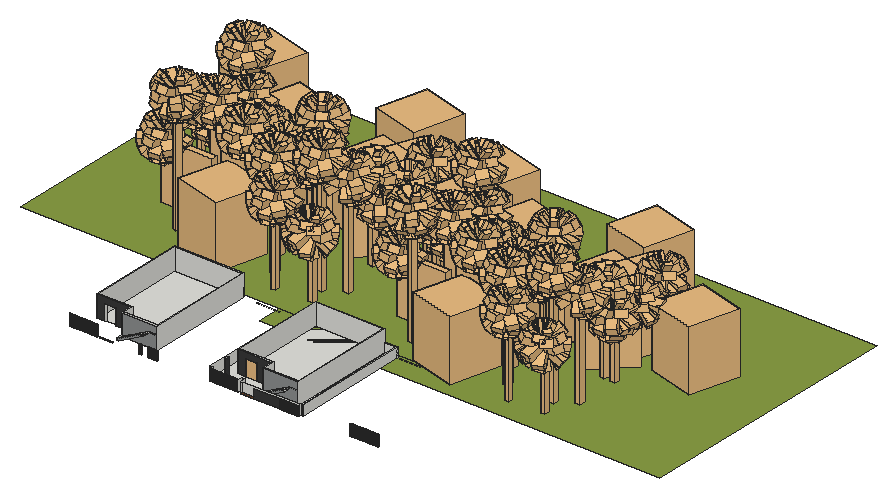
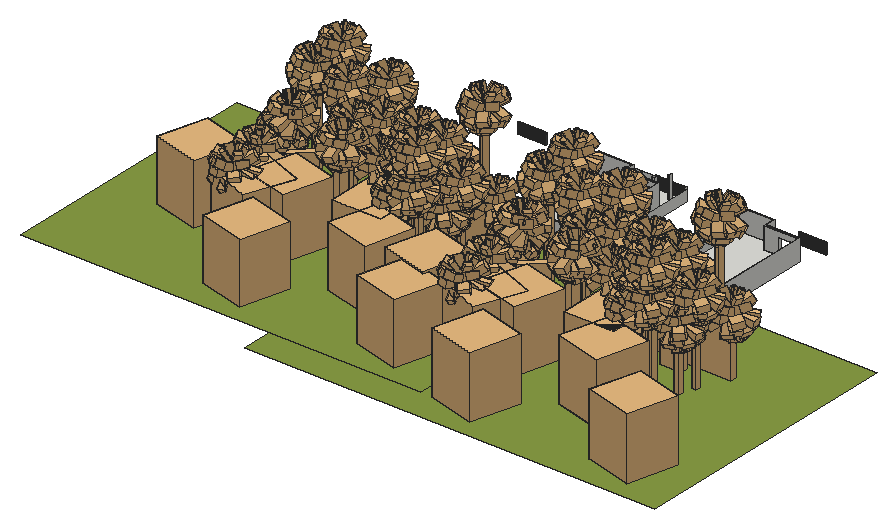
# SketchUp Ruby script. Lengths in inches.
U = 1.inch
M = Sketchup.active_model
def pt(a) = Geom::Point3d.new(a.map { |v| v * U })
def face(e, loops, mat)
  f = e.add_face(loops[0].map { |a| pt(a) })
  loops[1..].each { |l| e.add_face(l.map { |a| pt(a) }).erase! }
  f.material = f.back_material = mat if mat
  f
end
# faces: each face lists its corners as indices into pts; further lists are holes
def faces(e, pts, list, mat = nil) = list.each { |f| face(e, (f[0].is_a?(Array) ? f : [f]).map { |l| l.map { |i| pts[i] } }, mat) }
# xy, xz, yz: faces in a plane at the given z, y or x. An outline is a flat list of corners, or four numbers for a rectangle; further outlines are holes
def ring(l) = l.size == 4 ? [[l[0], l[1]], [l[2], l[1]], [l[2], l[3]], [l[0], l[3]]] : l.each_slice(2).to_a
def flat(e, list, mat, &to3) = list.each { |f| face(e, (f[0].is_a?(Array) ? f : [f]).map { |l| ring(l).map { |u, v| to3.(u, v) } }, mat) }
def xy(e, z, list, mat = nil) = flat(e, list, mat) { |x, y| [x, y, z] }
def xz(e, y, list, mat = nil) = flat(e, list, mat) { |x, z| [x, y, z] }
def yz(e, x, list, mat = nil) = flat(e, list, mat) { |y, z| [x, y, z] }
def lines(e, pts, list) = list.each { |a, b| e.add_line(pt(pts[a]), pt(pts[b])) }
# prism: a flat outline (further loops are holes) pulled along v
def prism(e, loops, v, mat = nil)
  f = face(e, loops, mat); d = Geom::Vector3d.new(v.map { |x| x * U })
  f.pushpull(f.normal.samedirection?(d) ? d.length : -d.length)
end
def box(e, o, s, mat = nil) = prism(e, [[o, [o[0] + s[0], o[1], o[2]], [o[0] + s[0], o[1] + s[1], o[2]], [o[0], o[1] + s[1], o[2]]]], [0, 0, s[2]], mat)
def at(x, y, z, deg = 0) = Geom::Transformation.translation(pt([x, y, z])) * Geom::Transformation.rotation(ORIGIN, Z_AXIS, deg.degrees)
def axes(o, x, y, z) = Geom::Transformation.new([*x, 0, *y, 0, *z, 0, *pt(o).to_a, 1])
def part(name) = M.definitions.add(name)
# library, detail: a bought-in or finely detailed component or shape, given as its bounding box
def library(name, o, s) = part(name).tap { |d| box(d.entities, o, s) }
def detail(e, o, s) = box(e.add_group.entities, o, s)
def put(e, d, t, mat = nil) = e.add_instance(d, t).tap { |i| i.material = mat if mat }
def group(e, t, mat = nil) = e.add_group.tap { |g| g.transformation = t; g.material = mat if mat }.entities
root = M.entities
M.materials.add("48,62,1").color = [75, 79, 82]
M.materials.add("COCOLUMBER1").color = [119, 109, 95]
M.materials.add("[Blacktop Old 02]").color = [143, 145, 145]
M.materials.add("[Color M07]").color = [58, 58, 58]
M.materials.add("[Grass Light Green]").color = [138, 158, 69]
M.materials.add("[Stone_Flagstone_Ashlar]").color = [175, 116, 102]
M.materials.add("[Wood Veneer 01]").color = [120, 70, 37]
M.materials.add("hpl-fundermax-sheets-500x500").color = [131, 93, 58]
c1 = part("Group\#60")
prism(c1.entities,[[[-0.75,0,69],[-0.75,0,68],[-0.75,-1.375,68],[-0.75,-1.375,4],[-0.75,0,4],[-0.75,0,3],[-0.75,-2.75,3],[-0.75,-2.75,69]]],[1.5,0,0])
c2 = part("Group\#59")
box(c2.entities,[0,-0.75,0],[0.75,0.75,72])
c3 = part("Group\#78")
xy(c3.entities,0,[[4.5,0,61.75,2],[62.25,0,120,2]])
xy(c3.entities,72,[[4.5,0,61.75,2],[62.25,0,120,2]])
xz(c3.entities,0,[[4.5,0,53.25,72],[54,0,57,72],[57.75,0,61.75,72],[62.25,0,66.25,72],[67,0,120,72]])
xz(c3.entities,0,[[57,0,57.75,72],[66.25,0,67,72]],"48,62,1")
xz(c3.entities,2,[[4.5,0,61.75,72],[62.25,0,120,72]])
yz(c3.entities,4.5,[[0,0,2,72]])
yz(c3.entities,61.75,[[0,0,2,72]])
yz(c3.entities,62.25,[[0,0,2,72]])
yz(c3.entities,120,[[0,0,2,72]])
put(c3.entities,c1,at(58,0,0))
put(c3.entities,c1,at(66,0,0))
put(c3.entities,c2,at(53.25,0,0),"48,62,1")
put(c3.entities,c2,at(49.5,0,0),"48,62,1")
put(c3.entities,c2,at(45.75,0,0),"48,62,1")
put(c3.entities,c2,at(42,0,0),"48,62,1")
put(c3.entities,c2,at(38.25,0,0),"48,62,1")
put(c3.entities,c2,at(34.5,0,0),"48,62,1")
put(c3.entities,c2,at(30.75,0,0),"48,62,1")
put(c3.entities,c2,at(27,0,0),"48,62,1")
put(c3.entities,c2,at(23.25,0,0),"48,62,1")
put(c3.entities,c2,at(19.5,0,0),"48,62,1")
put(c3.entities,c2,at(15.75,0,0),"48,62,1")
put(c3.entities,c2,at(12,0,0),"48,62,1")
put(c3.entities,c2,at(8.25,0,0),"48,62,1")
put(c3.entities,c2,at(4.5,0,0),"48,62,1")
put(c3.entities,c2,at(70,0,0),"48,62,1")
put(c3.entities,c2,at(73.75,0,0),"48,62,1")
put(c3.entities,c2,at(77.5,0,0),"48,62,1")
put(c3.entities,c2,at(81.25,0,0),"48,62,1")
put(c3.entities,c2,at(85,0,0),"48,62,1")
put(c3.entities,c2,at(88.75,0,0),"48,62,1")
put(c3.entities,c2,at(92.5,0,0),"48,62,1")
put(c3.entities,c2,at(96.25,0,0),"48,62,1")
put(c3.entities,c2,at(100,0,0),"48,62,1")
put(c3.entities,c2,at(103.75,0,0),"48,62,1")
put(c3.entities,c2,at(107.5,0,0),"48,62,1")
put(c3.entities,c2,at(111.25,0,0),"48,62,1")
put(c3.entities,c2,at(115,0,0),"48,62,1")
put(c3.entities,c2,at(119.25,0,0),"48,62,1")
c4 = library("door (1)",[38.93,25.48,0],[40,9.94,82.68])
c5 = library("Palm frond \#1",[-21.27,-0.38,-4.44],[74.64,151.68,26.05])
c6 = part("Palm frond cluster")
put(c6.entities,c5,axes([98.98,59.12,-6.6],[-0.57786,0.81614,0],[-0.81614,-0.57786,0],[0,0,1.8876]))
put(c6.entities,c5,axes([105.83,88.13,9.87],[-0.67944,-0.73373,0],[0.7249,-0.67126,-0.15471],[0.21427,-0.19842,1.86487]))
put(c6.entities,c5,axes([73.46,76.73,-6.83],[1,0,0],[0,0.99443,-0.10543],[0,0.19901,1.87708]))
c7 = part("Palm tree")
put(c7.entities,c5,axes([108.09,116.23,112.23],[0.60444,0.79634,0.02211],[-0.38669,0.31755,-0.86581],[-0.57427,0.42444,0.41215]))
put(c7.entities,c5,axes([136.99,132.05,110.62],[-0.9152,-0.38852,0.10706],[0.08408,-0.44389,-0.89213],[0.32496,-0.66577,0.36188]))
put(c7.entities,c5,axes([122.18,113.8,111.54],[0.08804,0.99481,0.05098],[-0.50379,0.08862,-0.85927],[-0.70852,0.0412,0.41966]))
put(c7.entities,c5,axes([127.99,125.91,114.12],[-0.30715,0.21543,0.04369],[-0.00716,-0.23041,1.0858],[0.26841,0.36655,0.07955]))
put(c7.entities,c5,axes([103.59,126.54,118.32],[0.96893,0.24682,0.01605],[-0.22321,0.84461,0.48663],[0.20112,-0.89679,1.64874]))
put(c7.entities,c5,axes([132.625,118.58,110.86],[-0.79198,0.60227,0.10017],[-0.36651,-0.33776,-0.86694],[-0.4026,-0.59638,0.40255]))
put(c7.entities,c5,axes([132.69,143.375,115.86],[-0.48474,-0.87071,0.083],[0.68927,-0.43869,-0.5766],[1.01639,-0.4196,1.53425]))
put(c7.entities,c6,axes([128.89,9.89,132.21],[0.59014,0.791,-0.16144],[-0.79634,0.60321,0.04452],[0.1326,0.10229,0.98588]))
put(c7.entities,c5,axes([110.58,141.22,117.1],[0.63855,-0.76931,0.0202],[0.63758,0.51415,-0.57371],[0.8135,0.71582,1.54559]))
put(c7.entities,c5,axes([124.78,146.64,115.88],[-0.11221,-0.99112,0.07129],[0.92652,-0.13028,-0.35296],[0.67787,0.04993,1.76097]))
put(c7.entities,c5,axes([122.51,149.42,117.04],[0.39103,-0.91975,0.03404],[0.19966,0.04866,-0.97866],[0.74078,0.32113,0.1671]))
put(c7.entities,c5,axes([109.625,140.35,117.99],[0.86054,-0.50891,0.02211],[0.4462,0.77402,0.44921],[-0.46382,-0.71105,1.68592]))
put(c7.entities,c5,axes([116.71,128.1875,118.1],[0.61604,-0.07661,0.00027],[0.03235,0.25679,-0.96593],[0.09819,0.79033,0.2134]),"COCOLUMBER1")
put(c7.entities,c5,axes([106.79,121.78,118.63],[0.90526,0.41496,-0.09122],[-0.38356,0.70587,-0.59551],[-0.34491,1.08363,1.50659]))
put(c7.entities,c5,axes([127.38,115.49,111.15],[-0.41996,0.90406,0.07938],[-0.48716,-0.15078,-0.8602],[-0.63133,-0.32974,0.41534]))
put(c7.entities,c5,axes([126.87,112.82,117.51],[-0.39428,0.9188,-0.01857],[-0.74747,-0.33238,-0.57517],[-1.00919,-0.40185,1.54373]))
put(c7.entities,c5,axes([136.51,114.68,116.54],[-0.8132,0.57038,0.11567],[-0.44883,-0.74115,0.49924],[0.69933,0.66833,1.62089]))
put(c7.entities,c5,axes([139.34,132.85,114.96],[-0.95658,-0.27018,0.10937],[0.1925,-0.86734,-0.45898],[0.41314,-0.78901,1.66428]))
put(c7.entities,c5,axes([114.58,111.42,117.76],[0.273,0.96044,0.05495],[-0.82871,0.20578,0.52048],[0.92224,-0.35418,1.60843]))
put(c7.entities,c6,axes([34.06,50.17,99.19],[1,0,0],[0,0.96593,0.25882],[0,-0.25882,0.96593]))
put(c7.entities,c5,axes([129.57,143.93,113.7],[-0.59821,-0.79634,0.08934],[0.41703,-0.40458,-0.81388],[0.56418,-0.37071,0.47337]))
put(c7.entities,c5,axes([130.72,144.4375,116.95],[-0.38164,-0.91976,0.09155],[0.8496,-0.31006,0.42666],[-0.68716,0.45418,1.6984]))
put(c7.entities,c5,axes([131.04,111.78,119.35],[-0.80044,0.5994,0.00413],[-0.42618,-0.56425,-0.7071],[-0.79563,-1.07169,1.33472]))
put(c7.entities,c5,axes([110.2,144.05,126.35],[0.60643,-0.7943,0.03632],[0.64903,0.52087,0.55448],[-0.86705,-0.59022,1.56936]))
put(c7.entities,c5,axes([142.64,131.42,116.29],[-0.95847,-0.25692,0.12379],[0.28487,-0.84195,0.45823],[-0.02548,0.8956,1.66141]))
put(c7.entities,c5,axes([119.45,118.27,117.33],[0.21648,0.59293,0.03228],[-0.46829,0.12335,0.87492],[0.90601,-0.35995,0.53567]))
put(c7.entities,c5,axes([117.27,113.7,118.04],[0.23506,0.97049,-0.05375],[-0.80388,0.16302,-0.57201],[-1.03133,0.33537,1.54496]))
put(c7.entities,c5,axes([111.15,130.86,117.79],[0.59448,-0.21434,0.01115],[0.17045,0.51639,0.83922],[-0.32671,-0.8747,0.60458]))
put(c7.entities,c5,axes([131.22,120.64,116.67],[-0.51397,0.3605,0.07311],[-0.2051,-0.46687,0.86021],[0.60585,0.75173,0.55245]))
put(c7.entities,c5,axes([124.93,138.67,117.02],[-0.21153,-0.59293,0.0562],[0.56288,-0.12335,0.81728],[-0.84066,0.35995,0.63331]))
put(c7.entities,c5,axes([125.97,109.88,116.19],[-0.24621,0.96375,0.10281],[-0.94431,-0.21463,-0.24942],[-0.41209,-0.29916,1.81761]))
put(c7.entities,c5,axes([112.49,114.18,118.67],[0.68775,0.72163,-0.07906],[-0.67912,0.60109,-0.4213],[-0.48416,0.64828,1.70539]))
c8 = part("Group\#557")
put(c8.entities,c7,axes([-0.04,31.24,176.27],[0.54092,-0.14494,0],[0.14494,0.54092,0],[0,0,0.56]),"[Stone_Flagstone_Ashlar]")
g1 = group(c8.entities,at(43.85,611.85,9.84))
detail(g1,[29.01,-534.03,-9.84],[20.18,17.89,236.22])
c9 = library("Group\#544",[280.3,-607.43,-9.84],[21.76,21.76,393.7])
c10 = part("Group\#559")
put(c10.entities,c7,axes([14.65,13.97,332.76],[0.56,0,0],[0,0.56,0],[0,0,0.56]),"[Stone_Flagstone_Ashlar]")
put(c10.entities,c9,at(-205.96,691.71,9.84))
c11 = library("Group\#545",[336.49,-607.32,-9.84],[23.63,23.62,472.44])
c12 = part("Group\#558")
put(c12.entities,c7,axes([14.65,13.97,408.41],[0.56,0,0],[0,0.56,0],[0,0,0.56]),"[Stone_Flagstone_Ashlar]")
put(c12.entities,c11,axes([-199.25,630.26,9.84],[0.8099,0,0],[0,0.92,0],[0,0,1]))
c13 = part("Group\#555")
put(c13.entities,c7,axes([14.65,13.97,257.21],[0.56,0,0],[0,0.56,0],[0,0,0.56]),"[Stone_Flagstone_Ashlar]")
g2 = group(c13.entities,at(-87.26,634.75,9.84))
detail(g2,[163.83,-557.35,-9.84],[17.02,18.12,316.37])
c14 = library("Coconut",[0,0,0],[6,6,6])
c15 = part("Group\#543")
detail(c15.entities,[126.53,-566.4375,-31.76],[21.43,21.47,314.96])
c16 = part("Group\#554")
put(c16.entities,c7,axes([14.65,13.97,253.0625],[0.56,0,0],[0,0.56,0],[0,0,0.56]),"[Stone_Flagstone_Ashlar]")
put(c16.entities,c15,at(-54.86,642.08,31.76))
c17 = library("Group\#560",[-31.7,-22.28,0],[197.44,197.48,245.38])
c18 = library("Group\#550",[-86.05,-583.93,-9.84],[105.44,25.13,372.44])
c19 = part("Group\#562")
put(c19.entities,c7,axes([14.65,13.97,296.01],[0.56,0,0],[0,0.56,0],[0,0,0.56]),"[Stone_Flagstone_Ashlar]")
put(c19.entities,c18,axes([86.81,656.51,9.45],[1,0,0],[0,1,0],[0,0,0.96]))
c20 = library("Group\#553",[-509.61,-583,-9.84],[198.33,25,224.95])
c21 = part("Group\#561")
put(c21.entities,c7,axes([14.65,13.97,164.57],[0.56,0,0],[0,0.56,0],[0,0,0.56]),"[Stone_Flagstone_Ashlar]")
put(c21.entities,c20,at(588.97,655.37,9.84))
c22 = library("Group\#551",[-201.8,-584.81,-9.84],[84.72,26.88,386.61])
c23 = library("Group\#552",[-284.02,-582.12,-9.84],[34.81,21.51,275.59])
c24 = part("LANDSCAPING+Coconut+Trees")
xy(c24.entities,0,[[-341.57,-22.89,1280.875,1071.24]],"[Grass Light Green]")
put(c24.entities,c8,at(644.25,162.65,0.08,-90))
put(c24.entities,c10,at(534.68,153.22,0.24))
put(c24.entities,c12,at(627.57,68.88,0.24))
g3 = group(c24.entities,at(441.06,62.32,0.24))
put(g3,c7,axes([14.65,13.97,334.3],[0.56,0,0],[0,0.56,0],[0,0,0.56]),"[Stone_Flagstone_Ashlar]")
g4 = group(g3,at(-161.71,683.51,9.84))
detail(g4,[235.77,-605.36,-9.84],[21.85,21.73,393.32])
put(c24.entities,c13,at(507.45,-17.04,0.04))
g5 = group(c24.entities,at(384.92,163.75,0.52))
put(g5,c7,axes([14.65,13.97,253.0625],[0.56,0,0],[0,0.56,0],[0,0,0.56]),"[Stone_Flagstone_Ashlar]")
put(g5,c14,axes([78.15,82.49,296.44],[0.8993,1.53487,-0.03138],[-1.51998,0.89531,0.23158],[0.21557,-0.09025,1.76378]))
put(g5,c14,axes([79.68,82.54,287.24],[0.80142,1.36782,-0.02796],[-1.35455,0.79787,0.20637],[0.1921,-0.08042,1.57182]))
put(g5,c14,axes([77.51,71.8,291.02],[0.8993,1.53487,-0.03138],[-1.51998,0.89531,0.23158],[0.21557,-0.09025,1.76378]))
put(g5,c14,axes([86.52,87.55,293.71],[1.04679,1.7866,-0.03652],[-1.76927,1.04215,0.26956],[0.25092,-0.10505,2.05306]))
put(g5,c14,axes([92.01,70.93,291.34],[1.26662,2.16178,-0.04419],[-2.14081,1.261,0.32616],[0.30361,-0.12711,2.4842]))
put(g5,c15,at(-54.86,642.08,31.76))
put(c24.entities,c16,at(322.43,275.42,0.52,75))
put(c24.entities,c17,at(215.66,444.05,0))
put(c24.entities,c19,at(219.87,194.55,1.28))
put(c24.entities,c21,at(-99.86,200.06,0.67))
g6 = group(c24.entities,at(71.46,249.51,0.63))
put(g6,c7,axes([14.65,13.97,325.99],[0.56,0,0],[0,0.56,0],[0,0,0.56]),"[Stone_Flagstone_Ashlar]")
put(g6,c22,at(259.05,660.06,9.84))
g7 = group(c24.entities,at(290.4,300.18,0.67))
put(g7,c7,axes([14.65,13.97,214.81],[0.56,0,0],[0,0.56,0],[0,0,0.56]),"[Stone_Flagstone_Ashlar]")
put(g7,c23,at(354.13,659.23,9.84))
put(c24.entities,c17,at(768.63,688.84,0,159))
put(c24.entities,c17,at(573.53,797.54,0,75))
put(c24.entities,c12,at(18.43,450.01,0.24))
put(c24.entities,c10,at(864.55,292.18,0.24,180))
put(c24.entities,c8,at(695.7,287.05,0.08))
put(c24.entities,c8,at(135.65,408.5625,0.08))
put(c24.entities,c21,at(771.29,622.71,0.67,-134.5))
put(c24.entities,c8,at(664.4,571.51,0.08))
put(c24.entities,c19,at(563.8125,499.28,1.28,140.1))
put(c24.entities,c13,at(450.29,232.17,0.04))
put(c24.entities,c13,at(-49.04,312.68,0.04))
put(c24.entities,c13,at(52.82,431.375,0.04))
put(c24.entities,c17,at(259.5,238.44,0,-105))
put(c24.entities,c17,at(533.19,658.43,0,-105))
put(c24.entities,c8,at(-26.35,370.51,0.08))
put(c24.entities,c17,at(-48.71,797.54,0,75))
put(c24.entities,c17,at(238.42,585.39,0,75))
put(c24.entities,c17,at(891.93,658.43,0,-105))
put(c24.entities,c12,at(220.5,234.49,0.24,165))
put(c24.entities,c16,at(795.86,275.42,0.52,75))
xy(root,5.875,[[1216.78,300.25,1219.26,301],[1219.97,300.25,1222.44,301],[1223.16,300.25,1225.63,301],[1226.35,300.25,1228.82,301],[1264.6,300.25,1267.07,301],
  [1267.78,300.25,1270.26,301],[1270.97,300.25,1273.44,301],[1274.16,300.25,1276.63,301],[1277.35,300.25,1279.82,301],[2003.16,300.25,2005.63,301],
  [2006.35,300.25,2008.82,301],[2009.53,300.25,2012.01,301],[2012.72,300.25,2015.19,301],[2015.91,300.25,2018.38,301],[2019.1,300.25,2021.57,301],
  [2022.28,300.25,2024.76,301],[2025.47,300.25,2027.94,301],[2028.66,300.25,2031.13,301],[2031.85,300.25,2034.32,301],[2035.03,300.25,2037.51,301],
  [2038.22,300.25,2040.69,301],[2041.41,300.25,2043.88,301],[2044.6,300.25,2047.07,301],[2047.78,300.25,2050.26,301],[2050.97,300.25,2053.44,301],
  [2054.16,300.25,2056.63,301],[2057.35,300.25,2059.82,301],[2060.53,300.25,2063.01,301],[2063.72,300.25,2066.19,301],[2066.91,300.25,2069.38,301],
  [2070.1,300.25,2072.57,301],[2073.22,300.25,2075.69,301],[2076.35,300.25,2078.82,301],[2079.47,300.25,2081.94,301],[2082.6,300.25,2085.07,301],
  [2085.72,300.25,2088.19,301],[2088.85,300.25,2091.32,301],[2091.97,300.25,2094.44,301],[2095.1,300.25,2097.57,301],[2098.22,300.25,2100.69,301],
  [2101.35,300.25,2103.82,301],[2104.47,300.25,2106.65,301],[[1609.83,301,1768.51,301,1768.51,327.09,1784.63,327.09,1784.63,308.75,2106.65,308.75,2106.65,315.3125,2114.96,315.3125,2114.96,969.375,2046.96,969.375,2046.96,371.33,1859.33,371.33,1859.33,335.33,1847.4,335.33,1847.4,431.33,1770.18,431.33,1770.18,440.27,1708.43,440.27,1708.43,431.33,1661.09,431.33,1661.09,952.09,1594.84,952.09,1594.84,321.97,1609.83,321.97],[1666.35,334.62,1673.73,350.3]],[1784.63,301,2106.65,308.75],[2114.96,315.3125,2120.96,969.375],
  [1061.03,335.33,1061.03,431.33,983.8,431.33,983.8,440.27,1067.03,440.27,1067.03,379.21,1255.32,379.21,1255.32,970.67,879.98,970.67,879.98,440.27,922.05,440.27,922.05,431.33,874.71,431.33,874.71,975.9375,1260.59,975.9375,1260.59,371.33,1072.95,371.33,1072.95,335.33],[1847.4,335.33,1847.4,431.33,1770.18,431.33,1770.18,440.27,1853.4,440.27,1853.4,379.21,2041.7,379.21,2041.7,970.67,1666.35,970.67,1666.35,440.27,1708.43,440.27,1708.43,431.33,1661.09,431.33,1661.09,975.9375,2046.96,975.9375,2046.96,371.33,1859.33,371.33,1859.33,335.33],[1067.03,379.21,1255.32,379.21,1255.32,970.67,879.98,970.67,879.98,440.27,1067.03,440.27],[1853.4,379.21,2041.7,379.21,2041.7,970.67,1666.35,970.67,1666.35,440.27,1853.4,440.27],[1334.59,969.375,1460.84,975.9375],
  [2046.96,969.375,2114.96,975.9375],[2114.96,969.375,2120.96,975.9375],[2120.96,969.375,2247.21,975.9375]])
xz(root,300.25,[[1216.78,5.875,1219.26,54.66],[1219.97,5.875,1222.44,54.66],[1223.16,5.875,1225.63,54.66],[1226.35,5.875,1228.82,54.66],[1264.6,5.875,1267.07,54.66],
  [1267.78,5.875,1270.26,54.66],[1270.97,5.875,1273.44,54.66],[1274.16,5.875,1276.63,54.66],[1277.35,5.875,1279.82,54.66],[2003.16,5.875,2005.63,54.66],
  [2006.35,5.875,2008.82,54.66],[2009.53,5.875,2012.01,54.66],[2012.72,5.875,2015.19,54.66],[2015.91,5.875,2018.38,54.66],[2019.1,5.875,2021.57,54.66],
  [2022.28,5.875,2024.76,54.66],[2025.47,5.875,2027.94,54.66],[2028.66,5.875,2031.13,54.66],[2031.85,5.875,2034.32,54.66],[2035.03,5.875,2037.51,54.66],
  [2038.22,5.875,2040.69,54.66],[2041.41,5.875,2043.88,54.66],[2044.6,5.875,2047.07,54.66],[2047.78,5.875,2050.26,54.66],[2050.97,5.875,2053.44,54.66],
  [2054.16,5.875,2056.63,54.66],[2057.35,5.875,2059.82,54.66],[2060.53,5.875,2063.01,54.66],[2063.72,5.875,2066.19,54.66],[2066.91,5.875,2069.38,54.66],
  [2070.1,5.875,2072.57,54.66],[2073.22,5.875,2075.69,54.66],[2076.35,5.875,2078.82,54.66],[2079.47,5.875,2081.94,54.66],[2082.6,5.875,2085.07,54.66],
  [2085.72,5.875,2088.19,54.66],[2088.85,5.875,2091.32,54.66],[2091.97,5.875,2094.44,54.66],[2095.1,5.875,2097.57,54.66],[2098.22,5.875,2100.69,54.66],
  [2101.35,5.875,2103.82,54.66],[2104.47,5.875,2106.65,54.66]],"[Color M07]")
xz(root,301,[[1320.28,5.875,1320.57,54.66],[2106.65,5.875,2106.94,54.66]])
xz(root,301,[[1283.01,5.875,1283.72,54.66],[1286.19,5.875,1286.85,54.66],[1289.32,5.875,1289.97,54.66],[1292.44,5.875,1293.1,54.66],[1295.57,5.875,1296.22,54.66],
  [1298.69,5.875,1299.35,54.66],[1301.82,5.875,1302.47,54.66],[1304.94,5.875,1305.6,54.66],[1308.07,5.875,1308.72,54.66],[1311.19,5.875,1311.85,54.66],
  [1314.32,5.875,1314.97,54.66],[1856.87,5.875,2003.16,54.66],[2005.63,5.875,2006.35,54.66],[2008.82,5.875,2009.53,54.66],[2012.01,5.875,2012.72,54.66],
  [2015.19,5.875,2015.91,54.66],[2018.38,5.875,2019.1,54.66],[2021.57,5.875,2022.28,54.66],[2024.76,5.875,2025.47,54.66],[2027.94,5.875,2028.66,54.66],
  [2031.13,5.875,2031.85,54.66],[2034.32,5.875,2035.03,54.66],[2037.51,5.875,2038.22,54.66],[2040.69,5.875,2041.41,54.66],[2043.88,5.875,2044.6,54.66],
  [2047.07,5.875,2047.78,54.66],[2050.26,5.875,2050.97,54.66],[2053.44,5.875,2054.16,54.66],[2056.63,5.875,2057.35,54.66],[2059.82,5.875,2060.53,54.66],
  [2063.01,5.875,2063.72,54.66],[2066.19,5.875,2066.91,54.66],[2069.38,5.875,2070.1,54.66],[2072.57,5.875,2073.22,54.66],[2075.69,5.875,2076.35,54.66],
  [2078.82,5.875,2079.47,54.66],[2081.94,5.875,2082.6,54.66],[2085.07,5.875,2085.72,54.66],[2088.19,5.875,2088.85,54.66],[2091.32,5.875,2091.97,54.66],
  [2094.44,5.875,2095.1,54.66],[2097.57,5.875,2098.22,54.66],[2100.69,5.875,2101.35,54.66],[2103.82,5.875,2104.47,54.66]],"[Color M07]")
xz(root,301,[[998.26,5.875,1070.49,13.04],[1784.63,5.875,1856.87,13.04]],"[Wood Veneer 01]")
xz(root,308.75,[[1784.63,5.875,2106.65,62.25]])
xz(root,315.3125,[[2106.65,5.875,2106.65,62.25,2120.96,62.25,2120.96,58.8125,2114.96,58.8125,2114.96,5.875],[2114.96,5.875,2120.96,58.8125]])
xz(root,321.97,[[1594.84,5.875,1609.83,65.875]])
xz(root,327.09,[[1768.51,5.875,1784.63,65.875]])
xz(root,334.62,[[1666.35,5.875,1673.73,125.875]],"[Color M07]")
xz(root,335.33,[[1061.03,5.875,1072.95,5.875,1217.03,77.875,1193.03,77.875,1193.03,71.875,1181.03,71.875,1181.03,65.875,1169.03,65.875,1169.03,59.875,1157.03,59.875,1157.03,53.875,1145.03,53.875,1145.03,47.875,1133.03,47.875,1133.03,41.875,1121.03,41.875,1121.03,35.875,1109.03,35.875,1109.03,29.875,1097.03,29.875,1097.03,23.875,1085.03,23.875,1085.03,17.875,1073.03,17.875,1073.03,11.875,1061.03,11.875],[1847.4,5.875,1859.33,5.875,2003.4,77.875,1979.4,77.875,1979.4,71.875,1967.4,71.875,1967.4,65.875,1955.4,65.875,1955.4,59.875,1943.4,59.875,1943.4,53.875,1931.4,53.875,1931.4,47.875,1919.4,47.875,1919.4,41.875,1907.4,41.875,1907.4,35.875,1895.4,35.875,1895.4,29.875,1883.4,29.875,1883.4,23.875,1871.4,23.875,1871.4,17.875,1859.4,17.875,1859.4,11.875,1847.4,11.875]],"[Blacktop Old 02]")
xz(root,350.3,[[1666.35,5.875,1673.73,125.875]])
xz(root,371.33,[[1072.95,5.875,1260.59,5.875,1260.59,125.875,1061.03,125.875,1061.03,11.875,1073.03,11.875,1073.03,17.875,1085.03,17.875,1085.03,23.875,1097.03,23.875,1097.03,29.875,1109.03,29.875,1109.03,35.875,1121.03,35.875,1121.03,41.875,1133.03,41.875,1133.03,47.875,1145.03,47.875,1145.03,53.875,1157.03,53.875,1157.03,59.875,1169.03,59.875,1169.03,65.875,1181.03,65.875,1181.03,71.875,1193.03,71.875,1193.03,77.875,1205.03,77.875,1205.03,83.875,1253.03,83.875,1253.03,77.875,1217.03,77.875],[1859.33,5.875,2046.96,5.875,2046.96,125.875,1847.4,125.875,1847.4,11.875,1859.4,11.875,1859.4,17.875,1871.4,17.875,1871.4,23.875,1883.4,23.875,1883.4,29.875,1895.4,29.875,1895.4,35.875,1907.4,35.875,1907.4,41.875,1919.4,41.875,1919.4,47.875,1931.4,47.875,1931.4,53.875,1943.4,53.875,1943.4,59.875,1955.4,59.875,1955.4,65.875,1967.4,65.875,1967.4,71.875,1979.4,71.875,1979.4,77.875,1991.4,77.875,1991.4,83.875,2039.4,83.875,2039.4,77.875,2003.4,77.875]],"[Blacktop Old 02]")
xz(root,379.21,[[1067.03,5.875,1255.32,125.875],[1853.4,5.875,2041.7,125.875]])
xz(root,431.33,[[874.71,5.875,922.05,5.875,922.05,94.0625,983.8,94.0625,983.8,5.875,1061.03,5.875,1061.03,125.875,874.71,125.875],[1661.09,5.875,1708.43,5.875,1708.43,94.0625,1770.18,94.0625,1770.18,5.875,1847.4,5.875,1847.4,125.875,1661.09,125.875]],"[Color M07]")
xz(root,440.27,[[879.98,5.875,879.98,125.875,1067.03,125.875,1067.03,5.875,983.8,5.875,983.8,94.0625,922.05,94.0625,922.05,5.875],[1666.35,5.875,1666.35,125.875,1853.4,125.875,1853.4,5.875,1770.18,5.875,1770.18,94.0625,1708.43,94.0625,1708.43,5.875]])
xz(root,952.09,[[1594.84,5.875,1661.09,65.875]])
xz(root,969.375,[[2046.96,5.875,2114.96,58.8125],[2114.96,5.875,2120.96,58.8125]])
xz(root,970.67,[[879.98,5.875,1255.32,125.875],[1666.35,5.875,2041.7,125.875]])
xz(root,975.9375,[[874.71,5.875,1260.59,125.875],[1661.09,5.875,2046.96,125.875],[2046.96,5.875,2114.96,58.8125],[2114.96,5.875,2120.96,58.8125]])
yz(root,874.71,[[431.33,5.875,431.33,125.875,975.9375,125.875,975.9375,65.875,952.09,65.875,952.09,5.875]])
yz(root,879.98,[[440.27,5.875,970.67,125.875]])
yz(root,922.05,[[431.33,5.875,440.27,94.0625]])
yz(root,983.8,[[431.33,5.875,440.27,94.0625]])
yz(root,1061.03,[[335.33,5.875,335.33,11.875,371.33,11.875,371.33,125.875,431.33,125.875,431.33,5.875]])
yz(root,1067.03,[[379.21,5.875,440.27,125.875]])
yz(root,1216.78,[[300.25,5.875,301,54.66]])
yz(root,1219.26,[[300.25,5.875,301,54.66]])
yz(root,1219.97,[[300.25,5.875,301,54.66]])
yz(root,1222.44,[[300.25,5.875,301,54.66]])
yz(root,1223.16,[[300.25,5.875,301,54.66]])
yz(root,1225.63,[[300.25,5.875,301,54.66]])
yz(root,1226.35,[[300.25,5.875,301,54.66]])
yz(root,1228.82,[[300.25,5.875,301,54.66]])
yz(root,1255.32,[[379.21,5.875,970.67,125.875]])
yz(root,1260.59,[[371.33,5.875,969.375,5.875,969.375,58.8125,975.9375,58.8125,975.9375,125.875,371.33,125.875]])
yz(root,1264.6,[[300.25,5.875,301,54.66]])
yz(root,1267.07,[[300.25,5.875,301,54.66]])
yz(root,1267.78,[[300.25,5.875,301,54.66]])
yz(root,1270.26,[[300.25,5.875,301,54.66]])
yz(root,1270.97,[[300.25,5.875,301,54.66]])
yz(root,1273.44,[[300.25,5.875,301,54.66]])
yz(root,1274.16,[[300.25,5.875,301,54.66]])
yz(root,1276.63,[[300.25,5.875,301,54.66]])
yz(root,1279.82,[[300.25,5.875,301,54.66]])
yz(root,1299.35,[[300.25,5.875,301,54.66]])
yz(root,1301.82,[[300.25,5.875,301,54.66]])
yz(root,1304.94,[[300.25,5.875,301,54.66]])
yz(root,1305.6,[[300.25,5.875,301,54.66]])
yz(root,1308.07,[[300.25,5.875,301,54.66]])
yz(root,1308.72,[[300.25,5.875,301,54.66]])
yz(root,1594.84,[[321.97,5.875,952.09,65.875]])
yz(root,1609.83,[[301,5.875,321.97,65.875]])
yz(root,1661.09,[[431.33,5.875,431.33,125.875,975.9375,125.875,975.9375,65.875,952.09,65.875,952.09,5.875],[952.09,5.875,975.9375,65.875]])
yz(root,1666.35,[[334.62,5.875,350.3,125.875],[440.27,5.875,970.67,125.875]])
yz(root,1673.73,[[334.62,5.875,350.3,125.875]],"[Color M07]")
yz(root,1708.43,[[431.33,5.875,440.27,94.0625]])
yz(root,1768.51,[[301,5.875,327.09,65.875]])
yz(root,1770.18,[[431.33,5.875,440.27,94.0625]])
yz(root,1784.63,[[301,5.875,308.75,62.25],[308.75,5.875,327.09,5.875,327.09,65.875,301,65.875,301,62.25,308.75,62.25]])
yz(root,1847.4,[[335.33,5.875,335.33,11.875,371.33,11.875,371.33,125.875,431.33,125.875,431.33,5.875]])
yz(root,1853.4,[[379.21,5.875,440.27,125.875]])
yz(root,2003.16,[[300.25,5.875,301,54.66]])
yz(root,2005.63,[[300.25,5.875,301,54.66]])
yz(root,2006.35,[[300.25,5.875,301,54.66]])
yz(root,2008.82,[[300.25,5.875,301,54.66]])
yz(root,2009.53,[[300.25,5.875,301,54.66]])
yz(root,2012.01,[[300.25,5.875,301,54.66]])
yz(root,2012.72,[[300.25,5.875,301,54.66]])
yz(root,2015.19,[[300.25,5.875,301,54.66]])
yz(root,2015.91,[[300.25,5.875,301,54.66]])
yz(root,2018.38,[[300.25,5.875,301,54.66]])
yz(root,2019.1,[[300.25,5.875,301,54.66]])
yz(root,2021.57,[[300.25,5.875,301,54.66]])
yz(root,2022.28,[[300.25,5.875,301,54.66]])
yz(root,2024.76,[[300.25,5.875,301,54.66]])
yz(root,2025.47,[[300.25,5.875,301,54.66]])
yz(root,2027.94,[[300.25,5.875,301,54.66]])
yz(root,2028.66,[[300.25,5.875,301,54.66]])
yz(root,2031.13,[[300.25,5.875,301,54.66]])
yz(root,2031.85,[[300.25,5.875,301,54.66]])
yz(root,2034.32,[[300.25,5.875,301,54.66]])
yz(root,2035.03,[[300.25,5.875,301,54.66]])
yz(root,2037.51,[[300.25,5.875,301,54.66]])
yz(root,2038.22,[[300.25,5.875,301,54.66]])
yz(root,2040.69,[[300.25,5.875,301,54.66]])
yz(root,2041.41,[[300.25,5.875,301,54.66]])
yz(root,2041.7,[[379.21,5.875,970.67,125.875]])
yz(root,2043.88,[[300.25,5.875,301,54.66]])
yz(root,2044.6,[[300.25,5.875,301,54.66]])
yz(root,2046.96,[[371.33,5.875,969.375,5.875,969.375,58.8125,975.9375,58.8125,975.9375,125.875,371.33,125.875]])
yz(root,2047.07,[[300.25,5.875,301,54.66]])
yz(root,2047.78,[[300.25,5.875,301,54.66]])
yz(root,2050.26,[[300.25,5.875,301,54.66]])
yz(root,2050.97,[[300.25,5.875,301,54.66]])
yz(root,2053.44,[[300.25,5.875,301,54.66]])
yz(root,2054.16,[[300.25,5.875,301,54.66]])
yz(root,2056.63,[[300.25,5.875,301,54.66]])
yz(root,2057.35,[[300.25,5.875,301,54.66]])
yz(root,2059.82,[[300.25,5.875,301,54.66]])
yz(root,2060.53,[[300.25,5.875,301,54.66]])
yz(root,2063.01,[[300.25,5.875,301,54.66]])
yz(root,2063.72,[[300.25,5.875,301,54.66]])
yz(root,2066.19,[[300.25,5.875,301,54.66]])
yz(root,2066.91,[[300.25,5.875,301,54.66]])
yz(root,2069.38,[[300.25,5.875,301,54.66]])
yz(root,2070.1,[[300.25,5.875,301,54.66]])
yz(root,2072.57,[[300.25,5.875,301,54.66]])
yz(root,2073.22,[[300.25,5.875,301,54.66]])
yz(root,2075.69,[[300.25,5.875,301,54.66]])
yz(root,2076.35,[[300.25,5.875,301,54.66]])
yz(root,2078.82,[[300.25,5.875,301,54.66]])
yz(root,2079.47,[[300.25,5.875,301,54.66]])
yz(root,2081.94,[[300.25,5.875,301,54.66]])
yz(root,2082.6,[[300.25,5.875,301,54.66]])
yz(root,2085.07,[[300.25,5.875,301,54.66]])
yz(root,2085.72,[[300.25,5.875,301,54.66]])
yz(root,2088.19,[[300.25,5.875,301,54.66]])
yz(root,2088.85,[[300.25,5.875,301,54.66]])
yz(root,2091.32,[[300.25,5.875,301,54.66]])
yz(root,2091.97,[[300.25,5.875,301,54.66]])
yz(root,2094.44,[[300.25,5.875,301,54.66]])
yz(root,2095.1,[[300.25,5.875,301,54.66]])
yz(root,2097.57,[[300.25,5.875,301,54.66]])
yz(root,2098.22,[[300.25,5.875,301,54.66]])
yz(root,2100.69,[[300.25,5.875,301,54.66]])
yz(root,2101.35,[[300.25,5.875,301,54.66]])
yz(root,2103.82,[[300.25,5.875,301,54.66]])
yz(root,2104.47,[[300.25,5.875,301,54.66]])
yz(root,2106.65,[[300.25,5.875,301,54.66],[308.75,5.875,315.3125,62.25]])
yz(root,2114.96,[[315.3125,5.875,969.375,58.8125],[969.375,5.875,975.9375,58.8125]])
yz(root,2120.96,[[315.3125,5.875,969.375,58.8125],[969.375,5.875,975.9375,58.8125]])
p = [[1072.95,371.33,5.875],[1217.03,371.33,77.875],[1217.03,335.33,77.875],[1072.95,335.33,5.875],[1859.33,371.33,5.875],[2003.4,371.33,77.875],
  [2003.4,335.33,77.875],[1859.33,335.33,5.875]]
faces(root,p,[[0,1,2,3],[4,5,6,7]])
put(root,c3,axes([1774.6875,305.75,5.875],[-1.37386,0,0],[0,1,0],[0,0,0.83333]),"hpl-fundermax-sheets-500x500")
put(root,c3,axes([988.3125,305.75,5.875],[-1.37386,0,0],[0,1,0],[0,0,0.83333]),"hpl-fundermax-sheets-500x500")
put(root,c3,axes([2555.0625,305.75,5.875],[-1.37386,0,0],[0,1,0],[0,0,0.83333]),"hpl-fundermax-sheets-500x500")
put(root,c4,axes([1648.33,403.11,5.875],[1.54375,0,0],[0,1,0],[0,0,1.06665]))
put(root,c24,axes([1913.81,886.79,5.875],[1.3776,0,0],[0,1.3776,0],[0,0,1.3776]))
put(root,c24,axes([481.61,1024.38,5.875],[1.41,0,0],[0,1.41,0],[0,0,1.41]))
